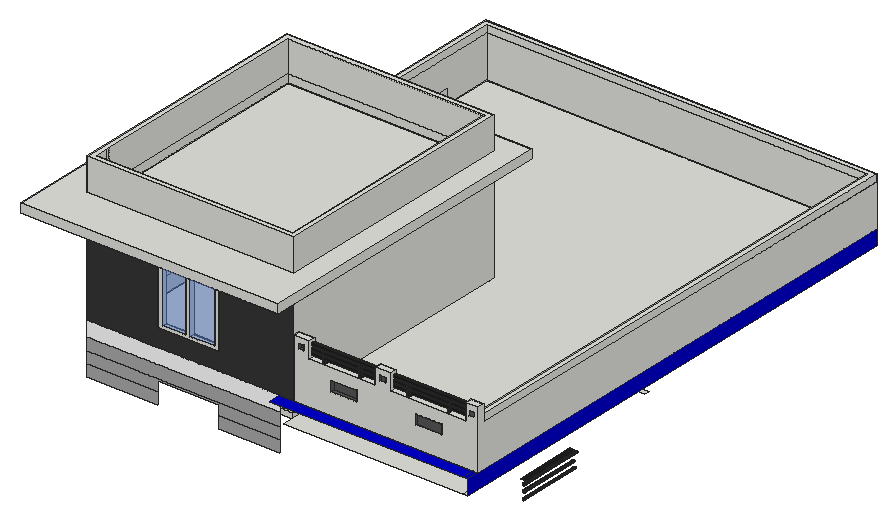
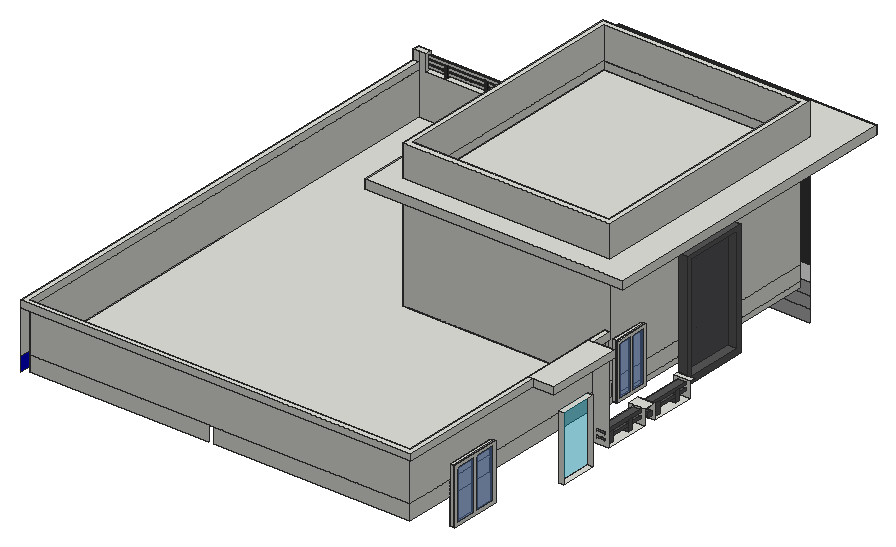
# SketchUp Ruby script. Lengths in inches.
U = 1.inch
M = Sketchup.active_model
def pt(a) = Geom::Point3d.new(a.map { |v| v * U })
def face(e, loops, mat)
  f = e.add_face(loops[0].map { |a| pt(a) })
  loops[1..].each { |l| e.add_face(l.map { |a| pt(a) }).erase! }
  f.material = f.back_material = mat if mat
  f
end
# faces: each face lists its corners as indices into pts; further lists are holes
def faces(e, pts, list, mat = nil) = list.each { |f| face(e, (f[0].is_a?(Array) ? f : [f]).map { |l| l.map { |i| pts[i] } }, mat) }
# xy, xz, yz: faces in a plane at the given z, y or x. An outline is a flat list of corners, or four numbers for a rectangle; further outlines are holes
def ring(l) = l.size == 4 ? [[l[0], l[1]], [l[2], l[1]], [l[2], l[3]], [l[0], l[3]]] : l.each_slice(2).to_a
def flat(e, list, mat, &to3) = list.each { |f| face(e, (f[0].is_a?(Array) ? f : [f]).map { |l| ring(l).map { |u, v| to3.(u, v) } }, mat) }
def xy(e, z, list, mat = nil) = flat(e, list, mat) { |x, y| [x, y, z] }
def xz(e, y, list, mat = nil) = flat(e, list, mat) { |x, z| [x, y, z] }
def yz(e, x, list, mat = nil) = flat(e, list, mat) { |y, z| [x, y, z] }
def lines(e, pts, list) = list.each { |a, b| e.add_line(pt(pts[a]), pt(pts[b])) }
# prism: a flat outline (further loops are holes) pulled along v
def prism(e, loops, v, mat = nil)
  f = face(e, loops, mat); d = Geom::Vector3d.new(v.map { |x| x * U })
  f.pushpull(f.normal.samedirection?(d) ? d.length : -d.length)
end
def box(e, o, s, mat = nil) = prism(e, [[o, [o[0] + s[0], o[1], o[2]], [o[0] + s[0], o[1] + s[1], o[2]], [o[0], o[1] + s[1], o[2]]]], [0, 0, s[2]], mat)
def at(x, y, z, deg = 0) = Geom::Transformation.translation(pt([x, y, z])) * Geom::Transformation.rotation(ORIGIN, Z_AXIS, deg.degrees)
def axes(o, x, y, z) = Geom::Transformation.new([*x, 0, *y, 0, *z, 0, *pt(o).to_a, 1])
def part(name) = M.definitions.add(name)
# library, detail: a bought-in or finely detailed component or shape, given as its bounding box
def library(name, o, s) = part(name).tap { |d| box(d.entities, o, s) }
def detail(e, o, s) = box(e.add_group.entities, o, s)
def put(e, d, t, mat = nil) = e.add_instance(d, t).tap { |i| i.material = mat if mat }
def group(e, t, mat = nil) = e.add_group.tap { |g| g.transformation = t; g.material = mat if mat }.entities
root = M.entities
M.materials.add("[Blinds Roman Hobbled Blue]").color = [81, 82, 87]
M.materials.add("[Color I06]").color = [0, 0, 204]
M.materials.add("[Color M00]").color = [255, 255, 255]
M.materials.add("[Color M03]").color = [170, 170, 170]
M.materials.add("[Color M06]").color = [86, 86, 86]
M.materials.add("[Color M08]").color = [30, 30, 30]
M.materials.add("[Slate Light Tile]").color = [54, 54, 54]
M.materials.add("[Translucent Glass Blue]").color = [100, 149, 237]
M.materials["[Translucent Glass Blue]"].alpha = 0.5
M.materials.add("[Translucent Glass Tinted]").color = [8, 201, 241]
M.materials["[Translucent Glass Tinted]"].alpha = 0.48
c1 = part("Group\#2")
xy(c1.entities,0,[[0,0,37.8125,5]])
xy(c1.entities,2.57,[[2.57,0,17.37,5],[19.91,0,35.24,5]])
xy(c1.entities,44.8,[[2.57,0,17.37,5],[19.91,0,35.24,5]])
xy(c1.entities,47.375,[[0,0,37.8125,5]])
xz(c1.entities,0,[[[0,0,37.8125,47.375],[19.91,2.57,35.24,44.8],[2.57,2.57,17.37,44.8]]])
xz(c1.entities,0,[[2.57,2.57,17.37,44.8],[19.91,2.57,35.24,44.8]],"[Translucent Glass Blue]")
xz(c1.entities,5,[[[0,0,37.8125,47.375],[19.91,2.57,35.24,44.8],[2.57,2.57,17.37,44.8]]])
yz(c1.entities,0,[[0,0,5,47.375]])
yz(c1.entities,2.57,[[0,2.57,5,44.8]])
yz(c1.entities,17.37,[[0,2.57,5,44.8]])
yz(c1.entities,19.91,[[0,2.57,5,44.8]])
yz(c1.entities,35.24,[[0,2.57,5,44.8]])
yz(c1.entities,37.8125,[[0,0,5,47.375]])
c2 = part("Group\#3")
xy(c2.entities,0,[[0,0,37.8125,5]])
xy(c2.entities,2.57,[[2.57,0,17.37,5],[19.91,0,35.24,5]])
xy(c2.entities,44.8,[[2.57,0,17.37,5],[19.91,0,35.24,5]])
xy(c2.entities,47.375,[[0,0,37.8125,5]])
xz(c2.entities,0,[[[0,0,37.8125,47.375],[19.91,2.57,35.24,44.8],[2.57,2.57,17.37,44.8]]])
xz(c2.entities,0,[[2.57,2.57,17.37,44.8],[19.91,2.57,35.24,44.8]],"[Translucent Glass Blue]")
xz(c2.entities,5,[[[0,0,37.8125,47.375],[19.91,2.57,35.24,44.8],[2.57,2.57,17.37,44.8]]])
yz(c2.entities,0,[[0,0,5,47.375]])
yz(c2.entities,2.57,[[0,2.57,5,44.8]])
yz(c2.entities,17.37,[[0,2.57,5,44.8]])
yz(c2.entities,19.91,[[0,2.57,5,44.8]])
yz(c2.entities,35.24,[[0,2.57,5,44.8]])
yz(c2.entities,37.8125,[[0,0,5,47.375]])
xy(root,365.83,[[59.3125,385.09,64.9375,426.22]])
xy(root,367,[[438.18,332.8125,486.18,338.8125]])
xy(root,368.47,[[364.5,332.8125,411.32,338.8125]])
xy(root,373.64,[[77.4375,500.02,83.4375,556.96]])
xy(root,375.04,[[[59.3125,248.07,77.4375,298.6],[63.67,286.08,72.73,290.83],[63.67,258.14,72.73,262.89]],[63.67,258.14,72.73,262.89],[63.67,286.08,72.73,290.83],[[59.3125,311.55,77.4375,362.77],[63.67,351.2,72.73,355.95],[63.67,324.83,72.73,329.58]],[63.67,324.83,72.73,329.58],
  [63.67,351.2,72.73,355.95]])
xy(root,380.88,[[64.33,248.07,73.2,362.77]],"[Color M06]")
xy(root,382.11,[[67.1875,241.6875,77.4375,241.87]])
xy(root,382.11,[[67.1875,166.06,77.4375,241.6875]],"[Color M06]")
xy(root,382.24,[[512.75,125.25,518.75,194.63]],"[Color M08]")
xy(root,384.01,[[64.33,248.07,73.2,362.77]],"[Color M06]")
xy(root,385.87,[[157.85,56.875,226.03,62.875]])
xy(root,387.19,[[64.33,248.07,73.2,362.77]],"[Color M06]")
xy(root,387.42,[[63.67,351.2,72.73,355.95]])
xy(root,387.48,[[63.67,324.83,72.73,329.58]])
xy(root,387.54,[[63.67,286.08,72.73,290.83]])
xy(root,387.79,[[63.67,258.14,72.73,262.89]])
xy(root,389.28,[[67.1875,171.71,77.4375,236.59]],"[Color M06]")
xy(root,390.32,[[64.33,248.07,73.2,362.77]],"[Color M06]")
xy(root,392.36,[[59.3125,241.6875,67.1875,241.6875,67.1875,241.87,77.4375,241.87,77.4375,248.07,59.3125,248.07],[59.3125,298.6,77.4375,311.55]])
xy(root,397,[[83.4375,62.875,304.75,332.8125]])
xy(root,398.88,[[77.4375,287.71,83.4375,327.77]])
xy(root,403,[[310.75,42.6875,512.75,332.8125],[512.75,42.6875,518.75,56.875],[83.4375,62.875,304.75,332.8125]])
xy(root,420,[[310.75,56.875,512.75,64.58],[310.75,64.58,512.75,64.58,512.75,613.125,83.4375,613.125,83.4375,338.8125,310.75,338.8125]])
xy(root,420,[[295.25,42.6875,512.75,56.875],[512.75,42.6875,518.75,56.875]],"[Color I06]")
xy(root,436.08,[[77.4375,500.02,83.4375,556.96]])
xy(root,438.77,[[59.3125,385.09,64.9375,426.22]])
xy(root,439.49,[[157.85,56.875,226.03,62.875]])
xy(root,444,[[352.48,56.875,382.17,61.5],[448.48,56.875,478.17,57.875]],"[Color M06]")
xy(root,455.5,[[352.48,56.875,382.17,61.5],[448.48,56.875,478.17,57.875]],"[Color M06]")
xy(root,461.44,[[77.4375,287.71,83.4375,327.77]])
xy(root,468,[[[328.01,56.875,402.58,64.58],[341.61,59.5,344.61,62.5],[382.55,59.5,385.55,62.5]],[[420.36,56.875,504.61,64.58],[436.8,59.5,439.8,62.5],[482.11,59.5,485.11,62.5]],[341.61,59.5,344.61,62.5],[382.55,59.5,385.55,62.5],[436.8,59.5,439.8,62.5],
  [482.11,59.5,485.11,62.5],[512.75,64.58,512.75,613.125,83.4375,613.125,83.4375,338.8125,77.4375,338.8125,77.4375,362.77,59.3125,362.77,59.3125,446.27,77.4375,446.27,77.4375,619.125,518.75,619.125,518.75,64.58],[53.8125,361.46,59.3125,447.64],[59.3125,361.46,77.4375,362.77],[59.3125,446.27,77.4375,447.64]])
xy(root,471.7,[[328.01,59.09,504.61,62.03]])
xy(root,474.15,[[316.02,56.875,322.27,61],[408.21,56.875,414.46,57.6875]],"[Color M06]")
xy(root,474.64,[[328.01,59.09,504.61,62.03]],"[Color M08]")
xy(root,475.875,[[512.75,64.58,518.75,64.58,518.75,619.125,77.4375,619.125,77.4375,446.27,83.4375,446.27,83.4375,613.125,512.75,613.125],[77.4375,338.8125,83.4375,362.77],[53.8125,361.46,77.4375,361.46,77.4375,362.77,83.4375,362.77,83.4375,446.27,77.4375,446.27,77.4375,447.64,53.8125,447.64]])
xy(root,476.51,[[328.01,59.09,512.75,62.03]])
xy(root,479.45,[[328.01,59.09,512.75,62.03]],"[Color M08]")
xy(root,480.4,[[316.02,56.875,322.27,61],[408.21,56.875,414.46,57.6875]],"[Color M06]")
xy(root,481.4375,[[482.11,59.5,485.11,62.5]])
xy(root,481.45,[[328.01,59.09,328.01,62.03,382.55,62.03,382.55,59.5,385.55,59.5,385.55,62.03,436.8,62.03,436.8,59.5,439.8,59.5,439.8,62.03,504.61,62.03,504.61,59.09],[382.55,59.5,385.55,62.03],[436.8,59.5,439.8,62.03],[382.55,62.03,385.55,62.5],[436.8,62.03,439.8,62.5]])
xy(root,481.6875,[[341.61,59.5,344.61,62.5]])
xy(root,484.39,[[328.01,59.09,504.61,62.03]],"[Color M08]")
xy(root,486.3125,[[310.75,56.875,328.01,64.58],[402.58,56.875,420.36,64.58],[504.61,56.875,518.75,64.58]])
xy(root,507.9,[[67.1875,171.71,77.4375,236.59]])
xy(root,512.67,[[67.1875,166.06,77.4375,241.87]],"[Color M06]")
xy(root,520.81,[[157.85,56.875,226.03,62.875]])
xy(root,536,[[83.4375,62.875,304.75,332.8125]])
xy(root,540,[[44.375,4,77.4375,361.5625],[77.4375,4,335.625,56.875],[77.4375,56.875,77.4375,338.8125,310.75,338.8125,310.75,332.8125,83.4375,332.8125,83.4375,62.875,304.75,62.875,304.75,332.8125,310.75,332.8125,310.75,56.875],[310.75,56.875,335.625,332.8125],[83.4375,62.875,304.75,332.8125],
  [310.75,332.8125,335.625,361.5625],[77.4375,338.8125,310.75,361.5625]])
xy(root,549.375,[[[44.375,4,335.625,361.5625],[77.4375,56.875,310.75,338.8125]],[77.4375,56.875,77.4375,338.8125,310.75,338.8125,310.75,332.8125,83.4375,332.8125,83.4375,62.875,304.75,62.875,304.75,332.8125,310.75,332.8125,310.75,56.875]])
xy(root,585.375,[[77.4375,56.875,310.75,56.875,310.75,332.8125,304.75,332.8125,304.75,62.875,83.4375,62.875,83.4375,332.8125,310.75,332.8125,310.75,338.8125,77.4375,338.8125]])
xz(root,4,[[44.375,540,335.625,549.375]])
xz(root,56.875,[[[310.75,420,518.75,420,518.75,486.3125,504.61,486.3125,504.61,468,420.36,468,420.36,486.3125,402.58,486.3125,402.58,468,328.01,468,328.01,486.3125,310.75,486.3125],[352.48,444,382.17,455.5],[448.48,444,478.17,455.5],[316.02,474.15,322.27,480.4],[408.21,474.15,414.46,480.4],[508.52,474.15,514.77,480.4]],[77.4375,549.375,310.75,585.375]])
xz(root,56.875,[[77.4375,403,295.25,420]],"[Color M00]")
xz(root,56.875,[[77.4375,361.63,157.85,375.01],[226.03,361.63,295.25,375.01],[77.4375,375.01,157.85,375.01,157.85,385.87,226.03,385.87,226.03,375.01,295.25,375.01,295.25,388.38,77.4375,388.38],[77.4375,388.38,295.25,403]],"[Color M03]")
xz(root,56.875,[[508.52,474.15,514.77,480.4]],"[Color M06]")
xz(root,56.875,[[[77.4375,420,310.75,540],[157.85,439.49,226.03,520.81]]],"[Slate Light Tile]")
xz(root,57.6875,[[408.21,474.15,414.46,480.4]],"[Color M06]")
xz(root,57.875,[[448.48,444,478.17,455.5]],"[Color M06]")
xz(root,59.09,[[328.01,471.7,504.61,474.64],[328.01,476.51,512.75,479.45],[328.01,481.45,504.61,484.39]],"[Color M08]")
xz(root,59.5,[[341.61,468,344.61,481.6875],[382.55,468,385.55,481.45],[436.8,468,439.8,481.45],[482.11,468,485.11,481.4375]],"[Color M08]")
xz(root,61,[[316.02,474.15,322.27,480.4]],"[Color M06]")
xz(root,61.5,[[352.48,444,382.17,455.5]],"[Color M06]")
xz(root,62.03,[[328.01,471.7,504.61,474.64],[328.01,476.51,512.75,479.45],[328.01,481.45,504.61,484.39]])
xz(root,62.5,[[341.61,468,344.61,481.6875],[382.55,468,385.55,481.45],[436.8,468,439.8,481.45],[482.11,468,485.11,481.4375]])
xz(root,62.875,[[83.4375,397,304.75,403],[83.4375,403,304.75,420],[[83.4375,420,304.75,536],[157.85,439.49,226.03,520.81]],[83.4375,536,304.75,540],[83.4375,540,304.75,549.375],
  [83.4375,549.375,304.75,585.375]])
xz(root,64.58,[[310.75,420,310.75,486.3125,328.01,486.3125,328.01,468,402.58,468,402.58,486.3125,420.36,486.3125,420.36,468,504.61,468,504.61,486.3125,512.75,486.3125,512.75,420],[512.75,468,518.75,475.875],[512.75,475.875,518.75,486.3125]])
xz(root,125.25,[[516.02,361.29,516.36,361.34,516.67,361.47,516.95,361.68,517.15,361.95,517.29,362.26,517.33,362.6,517.29,362.94,517.15,363.26,516.95,363.53,516.67,363.74,516.36,363.87,516.02,363.92,515.68,363.87,515.36,363.74,515.09,363.53,514.88,363.26,514.75,362.94,514.71,362.6,514.75,362.26,514.88,361.95,515.09,361.68,515.36,361.47,515.68,361.34],[516.02,368.85,516.36,368.9,516.67,369.03,516.95,369.24,517.15,369.51,517.29,369.83,517.33,370.17,517.29,370.51,517.15,370.82,516.95,371.09,516.67,371.3,516.36,371.43,516.02,371.48,515.68,371.43,515.36,371.3,515.09,371.09,514.88,370.82,514.75,370.51,514.71,370.17,514.75,369.83,514.88,369.51,515.09,369.24,515.36,369.03,515.68,368.9]])
xz(root,166.06,[[67.1875,382.11,77.4375,512.67]],"[Color M06]")
xz(root,171.71,[[67.1875,389.28,77.4375,507.9]],"[Color M06]")
xz(root,195.32,[[516.02,368.85,515.68,368.9,515.36,369.03,515.09,369.24,514.88,369.51,514.75,369.83,514.71,370.17,514.75,370.51,514.88,370.82,515.09,371.09,515.36,371.3,515.68,371.43,516.02,371.48,516.36,371.43,516.67,371.3,516.95,371.09,517.15,370.82,517.29,370.51,517.33,370.17,517.29,369.83,517.15,369.51,516.95,369.24,516.67,369.03,516.36,368.9]])
xz(root,197.19,[[516.02,361.29,515.68,361.34,515.36,361.47,515.09,361.68,514.88,361.95,514.75,362.26,514.71,362.6,514.75,362.94,514.88,363.26,515.09,363.53,515.36,363.74,515.68,363.87,516.02,363.92,516.36,363.87,516.67,363.74,516.95,363.53,517.15,363.26,517.29,362.94,517.33,362.6,517.29,362.26,517.15,361.95,516.95,361.68,516.67,361.47,516.36,361.34]])
xz(root,199.13,[[516.02,376.42,515.68,376.46,515.36,376.59,515.09,376.8,514.88,377.07,514.75,377.39,514.71,377.73,514.75,378.07,514.88,378.38,515.09,378.66,515.36,378.86,515.68,379,516.02,379.04,516.36,379,516.67,378.86,516.95,378.66,517.15,378.38,517.29,378.07,517.33,377.73,517.29,377.39,517.15,377.07,516.95,376.8,516.67,376.59,516.36,376.46]])
xz(root,236.59,[[67.1875,389.28,77.4375,507.9]],"[Color M06]")
xz(root,241.87,[[67.1875,382.11,77.4375,392.36]])
xz(root,241.87,[[67.1875,392.36,77.4375,512.67]],"[Color M06]")
xz(root,248.07,[[[59.3125,375.04,77.4375,392.36],[64.33,387.19,73.2,390.32],[64.33,380.88,73.2,384.01]],[64.33,380.88,73.2,384.01]])
xz(root,258.14,[[63.67,375.04,72.73,387.79]],"[Color M06]")
xz(root,262.89,[[63.67,375.04,72.73,387.79]],"[Color M06]")
xz(root,286.08,[[63.67,375.04,72.73,387.54]],"[Color M06]")
xz(root,287.71,[[77.4375,398.88,83.4375,461.44]])
xz(root,290.83,[[63.67,375.04,72.73,387.54]],"[Color M06]")
xz(root,298.6,[[59.3125,375.04,77.4375,392.36]])
xz(root,311.55,[[59.3125,375.04,77.4375,392.36]])
xz(root,324.83,[[63.67,375.04,72.73,387.48]],"[Color M06]")
xz(root,327.77,[[77.4375,398.88,83.4375,461.44]])
xz(root,329.58,[[63.67,375.04,72.73,387.48]],"[Color M06]")
xz(root,332.8125,[[83.4375,397,179.79,403],[179.79,397,194.09,403],[194.09,397,304.75,403],[83.4375,403,304.75,420],[83.4375,420,304.75,536],
  [83.4375,536,304.75,540],[83.4375,540,304.75,549.375],[83.4375,549.375,304.75,585.375]])
xz(root,338.8125,[[83.4375,403,304.75,420],[83.4375,420,83.4375,475.875,77.4375,475.875,77.4375,540,310.75,540,310.75,420],[77.4375,468,83.4375,475.875],[77.4375,549.375,310.75,585.375]])
xz(root,351.2,[[63.67,375.04,72.73,387.42]],"[Color M06]")
xz(root,355.95,[[63.67,375.04,72.73,387.42]],"[Color M06]")
xz(root,361.46,[[53.8125,468,77.4375,475.875]])
xz(root,361.5625,[[44.375,540,335.625,549.375]])
xz(root,362.77,[[[59.3125,375.04,77.4375,468],[64.33,380.88,73.2,384.01],[64.33,387.19,73.2,390.32]]])
xz(root,385.09,[[59.3125,365.83,64.9375,438.77]])
xz(root,426.22,[[59.3125,365.83,64.9375,438.77]])
xz(root,447.64,[[53.8125,468,77.4375,475.875]])
xz(root,500.02,[[77.4375,373.64,83.4375,436.08]])
xz(root,556.96,[[77.4375,373.64,83.4375,436.08]])
xz(root,613.125,[[83.4375,403,304.75,420],[310.75,403,512.75,420],[83.4375,420,512.75,468],[83.4375,468,512.75,475.875]])
xz(root,619.125,[[77.4375,468,518.75,475.875]])
yz(root,44.375,[[4,540,361.5625,549.375]])
yz(root,53.8125,[[361.46,468,447.64,475.875]])
yz(root,59.3125,[[302.34,381.29,307.53,386.48]],"[Color M06]")
yz(root,63.67,[[258.14,375.04,262.89,387.79],[286.08,375.04,290.83,387.54],[324.83,375.04,329.58,387.48],[351.2,375.04,355.95,387.42]],"[Color M06]")
yz(root,64.33,[[248.07,380.88,362.77,384.01],[248.07,387.19,362.77,390.32]],"[Color M06]")
yz(root,64.9375,[[385.09,365.83,426.22,438.77]],"[Translucent Glass Tinted]")
yz(root,67.1875,[[241.6875,382.11,241.87,392.36]])
yz(root,67.1875,[[[166.06,382.11,166.06,512.67,241.87,512.67,241.87,392.36,241.6875,392.36,241.6875,382.11],[171.71,389.28,236.59,507.9]]],"[Color M06]")
yz(root,72.73,[[258.14,375.04,262.89,387.79],[286.08,375.04,290.83,387.54],[324.83,375.04,329.58,387.48],[351.2,375.04,355.95,387.42]])
yz(root,73.2,[[248.07,380.88,362.77,384.01],[248.07,387.19,362.77,390.32]])
yz(root,77.4375,[[338.8125,468,361.46,475.875],[447.64,468,619.125,475.875],[56.875,549.375,338.8125,585.375]])
yz(root,77.4375,[[171.71,389.28,236.59,507.9]],"[Blinds Roman Hobbled Blue]")
yz(root,83.4375,[[500.02,373.64,556.96,403],[62.875,397,332.8125,397,332.8125,403,327.77,403,327.77,398.88,287.71,398.88,287.71,403,62.875,403],[287.71,398.88,327.77,403],[62.875,403,287.71,420],[287.71,403,327.77,420],
  [327.77,403,332.8125,420],[338.8125,403,500.02,420],[500.02,403,556.96,420],[556.96,403,613.125,420],[[62.875,420,287.71,420,287.71,461.44,327.77,461.44,327.77,420,332.8125,420,332.8125,536,62.875,536],[153.86,427.23,217.18,497.04]],
  [287.71,420,327.77,461.44],[338.8125,420,500.02,420,500.02,436.08,556.96,436.08,556.96,420,613.125,420,613.125,468,338.8125,468],[500.02,420,556.96,436.08],[338.8125,468,613.125,475.875],[62.875,536,75.44,540],
  [75.44,536,79.82,540],[79.82,536,332.8125,540],[62.875,540,75.44,549.375],[75.44,540,79.82,549.375],[79.82,540,332.8125,549.375],
  [62.875,549.375,75.44,585.375],[75.44,549.375,79.82,585.375],[79.82,549.375,332.8125,585.375]])
yz(root,157.85,[[56.875,439.49,62.875,520.81]])
yz(root,226.03,[[56.875,439.49,62.875,520.81]])
yz(root,304.75,[[62.875,397,332.8125,403],[62.875,403,332.8125,420],[62.875,420,332.8125,536],[62.875,536,332.8125,540],[62.875,540,332.8125,549.375],
  [62.875,549.375,332.8125,585.375]])
yz(root,310.75,[[56.875,420,64.58,486.3125],[64.58,420,338.8125,420,338.8125,540,56.875,540,56.875,486.3125,64.58,486.3125],[56.875,549.375,338.8125,585.375]])
yz(root,316.02,[[56.875,474.15,61,480.4]],"[Color M06]")
yz(root,322.27,[[56.875,474.15,61,480.4]],"[Color M06]")
yz(root,328.01,[[[56.875,468,64.58,486.3125],[59.09,471.7,62.03,474.64],[59.09,476.51,62.03,479.45],[59.09,481.45,62.03,484.39]],[59.09,476.51,62.03,479.45],[59.09,481.45,62.03,484.39]])
yz(root,335.625,[[4,540,361.5625,549.375]])
yz(root,341.61,[[59.5,468,62.5,481.6875]],"[Color M08]")
yz(root,344.61,[[59.5,468,62.5,481.6875]],"[Color M08]")
yz(root,352.48,[[56.875,444,61.5,455.5]],"[Color M06]")
yz(root,382.17,[[56.875,444,61.5,455.5]],"[Color M06]")
yz(root,382.55,[[59.5,468,62.5,481.45]],"[Color M08]")
yz(root,385.55,[[59.5,468,62.5,481.45]],"[Color M08]")
yz(root,402.58,[[56.875,468,64.58,486.3125]])
yz(root,408.21,[[56.875,474.15,57.6875,480.4]],"[Color M06]")
yz(root,414.46,[[56.875,474.15,57.6875,480.4]],"[Color M06]")
yz(root,420.36,[[56.875,468,64.58,486.3125]])
yz(root,436.8,[[59.5,468,62.5,481.45]],"[Color M08]")
yz(root,439.8,[[59.5,468,62.5,481.45]],"[Color M08]")
yz(root,448.48,[[56.875,444,57.875,455.5]],"[Color M06]")
yz(root,478.17,[[56.875,444,57.875,455.5]],"[Color M06]")
yz(root,482.11,[[59.5,468,62.5,481.4375]],"[Color M08]")
yz(root,485.11,[[59.5,468,62.5,481.4375]],"[Color M08]")
yz(root,504.61,[[[56.875,468,64.58,486.3125],[59.09,481.45,62.03,484.39],[59.09,471.7,62.03,474.64]]])
yz(root,512.75,[[338.8125,403,613.125,420],[64.58,420,613.125,468],[64.58,468,613.125,475.875],[59.09,476.51,62.03,479.45]])
yz(root,518.75,[[56.875,420,619.125,420,619.125,468,64.58,468,64.58,486.3125,56.875,486.3125],[64.58,468,619.125,475.875]])
yz(root,518.75,[[42.6875,403,619.125,420]],"[Color I06]")
p = [[515.68,125.25,361.34],[515.36,125.25,361.47],[515.36,197.19,361.47],[515.68,197.19,361.34],[516.02,125.25,361.29],[516.02,197.19,361.29],
  [516.36,125.25,361.34],[516.36,197.19,361.34],[516.67,125.25,361.47],[516.67,197.19,361.47],[515.09,125.25,361.68],[515.09,197.19,361.68],
  [516.95,125.25,361.68],[516.95,197.19,361.68],[514.88,125.25,361.95],[514.88,197.19,361.95],[517.15,125.25,361.95],[517.15,197.19,361.95],
  [514.75,125.25,362.26],[514.75,197.19,362.26],[517.29,125.25,362.26],[517.29,197.19,362.26],[514.71,125.25,362.6],[514.71,197.19,362.6],
  [517.33,125.25,362.6],[517.33,197.19,362.6],[514.75,125.25,362.94],[514.75,197.19,362.94],[517.29,125.25,362.94],[517.29,197.19,362.94],
  [514.88,125.25,363.26],[514.88,197.19,363.26],[517.15,125.25,363.26],[517.15,197.19,363.26],[515.09,125.25,363.53],[515.09,197.19,363.53],
  [516.95,125.25,363.53],[516.95,197.19,363.53],[515.36,125.25,363.74],[515.36,197.19,363.74],[516.67,125.25,363.74],[516.67,197.19,363.74],
  [515.68,125.25,363.87],[515.68,197.19,363.87],[516.36,125.25,363.87],[516.36,197.19,363.87],[516.02,125.25,363.92],[516.02,197.19,363.92],
  [515.68,125.25,368.9],[515.36,125.25,369.03],[515.36,195.32,369.03],[515.68,195.32,368.9],[516.02,125.25,368.85],[516.02,195.32,368.85],
  [516.36,125.25,368.9],[516.36,195.32,368.9],[516.67,125.25,369.03],[516.67,195.32,369.03],[515.09,125.25,369.24],[515.09,195.32,369.24],
  [516.95,125.25,369.24],[516.95,195.32,369.24],[514.88,125.25,369.51],[514.88,195.32,369.51],[517.15,125.25,369.51],[517.15,195.32,369.51],
  [514.75,125.25,369.83],[514.75,195.32,369.83],[517.29,125.25,369.83],[517.29,195.32,369.83],[514.71,125.25,370.17],[514.71,195.32,370.17],
  [517.33,125.25,370.17],[517.33,195.32,370.17],[514.75,125.25,370.51],[514.75,195.32,370.51],[517.29,125.25,370.51],[517.29,195.32,370.51],
  [514.88,125.25,370.82],[514.88,195.32,370.82],[517.15,125.25,370.82],[517.15,195.32,370.82],[515.09,125.25,371.09],[515.09,195.32,371.09],
  [516.95,125.25,371.09],[516.95,195.32,371.09],[515.36,125.25,371.3],[515.36,195.32,371.3],[516.67,125.25,371.3],[516.67,195.32,371.3],
  [515.68,125.25,371.43],[515.68,195.32,371.43],[516.36,125.25,371.43],[516.36,195.32,371.43],[516.02,125.25,371.48],[516.02,195.32,371.48],
  [516.02,125.25,376.42],[515.68,125.25,376.46],[515.68,199.13,376.46],[516.02,199.13,376.42],[516.36,125.25,376.46],[516.36,199.13,376.46],
  [515.36,125.25,376.59],[515.36,199.13,376.59],[516.67,125.25,376.59],[516.67,199.13,376.59],[515.09,125.25,376.8],[515.09,199.13,376.8],
  [516.95,125.25,376.8],[516.95,199.13,376.8],[514.88,125.25,377.07],[514.88,199.13,377.07],[517.15,125.25,377.07],[517.15,199.13,377.07],
  [514.75,125.25,377.39],[514.75,199.13,377.39],[517.29,125.25,377.39],[517.29,199.13,377.39],[514.71,125.25,377.73],[514.71,199.13,377.73],
  [517.33,125.25,377.73],[517.33,199.13,377.73],[514.75,125.25,378.07],[514.75,199.13,378.07],[517.29,125.25,378.07],[517.29,199.13,378.07],
  [514.88,125.25,378.38],[514.88,199.13,378.38],[517.15,125.25,378.38],[517.15,199.13,378.38],[515.09,125.25,378.66],[515.09,199.13,378.66],
  [516.95,125.25,378.66],[516.95,199.13,378.66],[515.36,125.25,378.86],[515.36,199.13,378.86],[516.67,125.25,378.86],[516.67,199.13,378.86],
  [515.68,125.25,379],[515.68,199.13,379],[516.36,125.25,379],[516.36,199.13,379],[516.02,125.25,379.04],[516.02,199.13,379.04],
  [310.75,338.8125,403],[310.75,338.8125,420],[304.75,332.8125,420],[310.75,332.8125,420],[83.4375,338.8125,420],[77.4375,338.8125,420],
  [77.4375,153.86,427.23],[83.4375,153.86,427.23],[77.4375,217.18,427.23],[83.4375,217.18,427.23],[77.4375,153.86,497.04],[83.4375,153.86,497.04],
  [77.4375,217.18,497.04],[83.4375,217.18,497.04],[77.4375,153.86,383.85],[83.4375,153.86,383.85],[77.4375,217.18,383.85],[83.4375,217.18,383.85],
  [77.4375,56.875,540],[77.4375,56.875,549.375]]
faces(root,p,[[0,1,2,3],[4,0,3,5],[6,4,5,7],[8,6,7,9],[1,10,11,2],[12,8,9,13],[10,14,15,11],[16,12,13,17],
  [14,18,19,15],[20,16,17,21],[18,22,23,19],[24,20,21,25],[22,26,27,23],[28,24,25,29],[26,30,31,27],[32,28,29,33],
  [30,34,35,31],[36,32,33,37],[34,38,39,35],[40,36,37,41],[38,42,43,39],[44,40,41,45],[42,46,47,43],[46,44,45,47],
  [48,49,50,51],[52,48,51,53],[54,52,53,55],[56,54,55,57],[49,58,59,50],[60,56,57,61],[58,62,63,59],[64,60,61,65],
  [62,66,67,63],[68,64,65,69],[66,70,71,67],[72,68,69,73],[70,74,75,71],[76,72,73,77],[74,78,79,75],[80,76,77,81],
  [78,82,83,79],[84,80,81,85],[82,86,87,83],[88,84,85,89],[86,90,91,87],[92,88,89,93],[90,94,95,91],[94,92,93,95],
  [96,97,98,99],[100,96,99,101],[97,102,103,98],[104,100,101,105],[102,106,107,103],[108,104,105,109],[106,110,111,107],[112,108,109,113],
  [110,114,115,111],[116,112,113,117],[114,118,119,115],[120,116,117,121],[118,122,123,119],[124,120,121,125],[122,126,127,123],[128,124,125,129],
  [126,130,131,127],[132,128,129,133],[130,134,135,131],[136,132,133,137],[134,138,139,135],[140,136,137,141],[138,142,143,139],[142,140,141,143]],"[Color M08]")
lines(root,p,[[144,145],[146,147],[148,149],[150,151],[152,153],[154,155],[156,157],[158,159],[160,161],[162,163]])
put(root,c1,axes([77.4375,556.96,373.64],[0,-1.50579,0],[0.41,0,0],[0,0,1.32058]))
put(root,c1,axes([77.4375,327.97,398.88],[0,-1.06467,0],[0.41,0,0],[0,0,1.32058]))
put(root,c2,axes([157.85,56.875,439.49],[1.80331,0,0],[0,1,0],[0,0,1.71636]))
